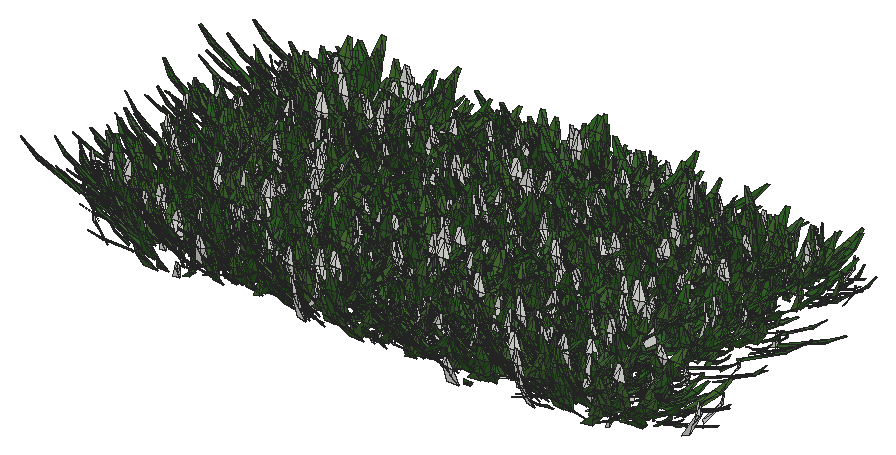
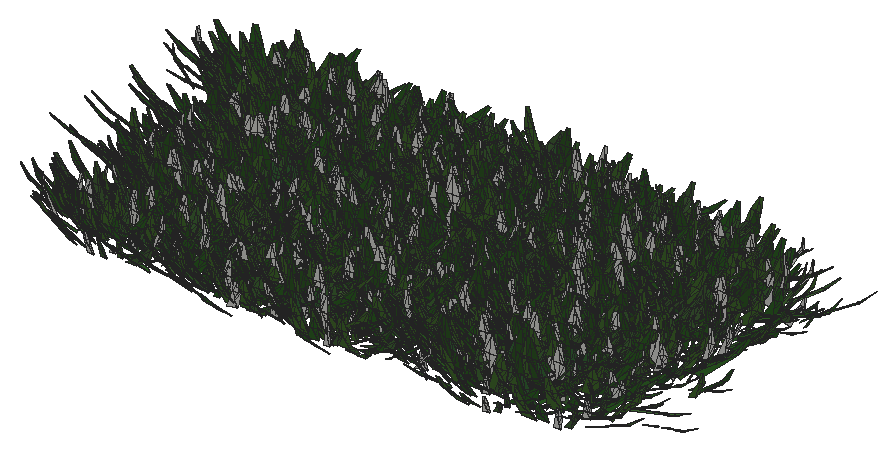
# SketchUp Ruby script. Lengths in inches.
U = 1.inch
M = Sketchup.active_model
def pt(a) = Geom::Point3d.new(a.map { |v| v * U })
def face(e, loops, mat)
  f = e.add_face(loops[0].map { |a| pt(a) })
  loops[1..].each { |l| e.add_face(l.map { |a| pt(a) }).erase! }
  f.material = f.back_material = mat if mat
  f
end
# faces: each face lists its corners as indices into pts; further lists are holes
def faces(e, pts, list, mat = nil) = list.each { |f| face(e, (f[0].is_a?(Array) ? f : [f]).map { |l| l.map { |i| pts[i] } }, mat) }
# xy, xz, yz: faces in a plane at the given z, y or x. An outline is a flat list of corners, or four numbers for a rectangle; further outlines are holes
def ring(l) = l.size == 4 ? [[l[0], l[1]], [l[2], l[1]], [l[2], l[3]], [l[0], l[3]]] : l.each_slice(2).to_a
def flat(e, list, mat, &to3) = list.each { |f| face(e, (f[0].is_a?(Array) ? f : [f]).map { |l| ring(l).map { |u, v| to3.(u, v) } }, mat) }
def xy(e, z, list, mat = nil) = flat(e, list, mat) { |x, y| [x, y, z] }
def xz(e, y, list, mat = nil) = flat(e, list, mat) { |x, z| [x, y, z] }
def yz(e, x, list, mat = nil) = flat(e, list, mat) { |y, z| [x, y, z] }
def lines(e, pts, list) = list.each { |a, b| e.add_line(pt(pts[a]), pt(pts[b])) }
# prism: a flat outline (further loops are holes) pulled along v
def prism(e, loops, v, mat = nil)
  f = face(e, loops, mat); d = Geom::Vector3d.new(v.map { |x| x * U })
  f.pushpull(f.normal.samedirection?(d) ? d.length : -d.length)
end
def box(e, o, s, mat = nil) = prism(e, [[o, [o[0] + s[0], o[1], o[2]], [o[0] + s[0], o[1] + s[1], o[2]], [o[0], o[1] + s[1], o[2]]]], [0, 0, s[2]], mat)
def at(x, y, z, deg = 0) = Geom::Transformation.translation(pt([x, y, z])) * Geom::Transformation.rotation(ORIGIN, Z_AXIS, deg.degrees)
def axes(o, x, y, z) = Geom::Transformation.new([*x, 0, *y, 0, *z, 0, *pt(o).to_a, 1])
def part(name) = M.definitions.add(name)
# library, detail: a bought-in or finely detailed component or shape, given as its bounding box
def library(name, o, s) = part(name).tap { |d| box(d.entities, o, s) }
def detail(e, o, s) = box(e.add_group.entities, o, s)
def put(e, d, t, mat = nil) = e.add_instance(d, t).tap { |i| i.material = mat if mat }
def group(e, t, mat = nil) = e.add_group.tap { |g| g.transformation = t; g.material = mat if mat }.entities
root = M.entities
M.materials.add("Material82").color = [68, 110, 58]
M.materials.add("Material83").color = [48, 90, 38]
M.materials.add("Material84").color = [68, 110, 48]
M.materials.add("Material85").color = [48, 90, 48]
M.materials.add("Material86").color = [58, 110, 58]
M.materials.add("Material87").color = [58, 90, 38]
M.materials.add("Material88").color = [68, 100, 58]
M.materials.add("Material89").color = [48, 100, 38]
c1 = part("grass00")
p = [[-0.6875,0.15,0],[-0.56,0.08,5.52],[-0.04,0.03,2.76],[0.48,-0.02,0],[0.35,-0.02,5.52],[-0.1,-0.14,5.52],
  [-0.12,0.65,8.37],[-0.42,0.65,8.37]]
faces(c1.entities,p,[[0,1,2,3],[3,2,4],[1,5,2],[5,4,2],[1,6,5],[4,5,6],[7,6,1]])
c2 = part("Group16\#1")
put(c2.entities,c1,axes([1.44,-0.61,-0.01],[0.05352,0.12609,0],[-0.10704,0.04543,0.07239],[0.06664,-0.02828,0.11628]),"Material85")
put(c2.entities,c1,axes([0.76,-0.15,-0.01],[0.04676,0.24062,0],[-0.23162,0.04501,0.06642],[0.0652,-0.01267,0.23595]),"Material82")
put(c2.entities,c1,axes([0.79,0.01,-0.01],[-0.00606,0.34651,0],[-0.34381,-0.00602,0.0432],[0.04319,0.00076,0.34386]))
put(c2.entities,c1,axes([1,0.23,-0.01],[-0.07192,0.31144,0],[-0.28722,-0.06632,0.1236],[0.12043,0.02781,0.29478]),"Material84")
put(c2.entities,c1,axes([1.66,0.77,-0.01],[-0.13828,0.29651,0],[-0.21551,-0.1005,0.22471],[0.20365,0.09498,0.23779]),"Material89")
put(c2.entities,c1,axes([0.6875,0.52,-0.01],[-0.18126,0.24051,0],[-0.22746,-0.17142,0.09788],[0.07817,0.05891,0.28481]),"Material84")
put(c2.entities,c1,axes([0.68,0.78,-0.01],[-0.215,0.18688,0],[-0.12385,-0.14248,0.21334],[0.13995,0.16101,0.18878]),"Material82")
put(c2.entities,c1,axes([0.56,1,-0.01],[-0.13756,0.07624,0],[-0.06159,-0.11112,0.0927],[0.04494,0.08108,0.12705]),"Material84")
put(c2.entities,c1,axes([0.2,0.64,-0.01],[-0.23729,0.07254,0],[-0.05711,-0.18681,0.153],[0.04473,0.14632,0.19535]),"Material89")
put(c2.entities,c1,axes([0.0625,0.72,-0.01],[-0.28874,0.02525,0],[-0.02179,-0.24916,0.14647],[0.01276,0.14591,0.25012]),"Material82")
put(c2.entities,c1,axes([-0.08,0.62,-0.01],[-0.34089,-0.04187,0],[0.03255,-0.26504,0.216],[-0.02633,0.21439,0.26703]),"Material89")
put(c2.entities,c1,axes([-0.34,0.98,-0.01],[-0.14314,-0.0493,0],[0.04397,-0.12769,0.06843],[-0.02228,0.0647,0.13505]),"Material89")
put(c2.entities,c1,axes([-0.87,1.45,-0.01],[-0.23488,-0.14114,0],[0.13761,-0.22901,0.06087],[-0.03135,0.05217,0.26717]))
put(c2.entities,c1,axes([-0.72,0.77,-0.01],[-0.14208,-0.13251,0],[0.07209,-0.0773,0.16301],[-0.11118,0.11922,0.1057]),"Material89")
put(c2.entities,c1,axes([-0.62,0.43,-0.01],[-0.14845,-0.21203,0],[0.18654,-0.13061,0.12304],[-0.10079,0.07057,0.22772]),"Material82")
put(c2.entities,c1,axes([-0.68,0.29,-0.01],[-0.13639,-0.32136,0],[0.31723,-0.13464,0.05579],[-0.05136,0.0218,0.34462]),"Material83")
put(c2.entities,c1,axes([-0.64,0.125,-0.01],[-0.0458,-0.23569,0],[0.22124,-0.043,0.08276],[-0.08124,0.01579,0.22538]),"Material86")
put(c2.entities,c1,axes([-1.6,-0.03,-0.01],[0.00576,-0.32897,0],[0.27526,0.00482,0.18018],[-0.18015,-0.00315,0.2753]),"Material84")
put(c2.entities,c1,axes([-1.36,-0.31,-0.01],[0.05718,-0.24765,0],[0.18172,0.04196,0.17267],[-0.16825,-0.03885,0.1865]),"Material89")
put(c2.entities,c1,axes([-1.54,-0.72,-0.01],[0.06537,-0.14017,0],[0.13555,0.06321,0.03939],[-0.0357,-0.01665,0.14956]))
put(c2.entities,c1,axes([-1.19,-0.9,-0.01],[0.09597,-0.12735,0],[0.11214,0.08451,0.07557],[-0.06035,-0.04548,0.14042]),"Material88")
put(c2.entities,c1,axes([-0.47,-0.54,-0.01],[0.11588,-0.10072,0],[0.0618,0.0711,0.12124],[-0.07953,-0.0915,0.0942]))
put(c2.entities,c1,axes([-0.47,-0.84,-0.01],[0.11927,-0.0661,0],[0.06603,0.11913,0.00646],[-0.00313,-0.00565,0.13621]),"Material84")
put(c2.entities,c1,axes([-0.38,-1.24,-0.01],[0.28037,-0.08571,0],[0.0618,0.20215,0.20315],[-0.05939,-0.19428,0.21139]),"Material88")
put(c2.entities,c1,axes([-0.06,-0.66,-0.01],[0.22719,-0.01987,0],[0.01247,0.14255,0.17758],[-0.01547,-0.17691,0.1431]),"Material87")
put(c2.entities,c1,axes([0.11,-0.89,-0.01],[0.14882,0.01828,0],[-0.01058,0.08611,0.12229],[0.01491,-0.12138,0.08676]),"Material85")
put(c2.entities,c1,axes([0.25,-0.72,-0.01],[0.20481,0.07053,0],[-0.06206,0.18022,0.10291],[0.03351,-0.0973,0.1906]),"Material85")
put(c2.entities,c1,axes([0.85,-1.42,-0.01],[0.16481,0.09904,0],[-0.09472,0.15762,0.05616],[0.02893,-0.04814,0.18389]),"Material84")
put(c2.entities,c1,axes([1.01,-1.09,-0.01],[0.21858,0.20385,0],[-0.17495,0.1876,0.15339],[0.10462,-0.11218,0.25652]),"Material89")
put(c2.entities,c1,axes([1.01,-0.71,-0.01],[0.08733,0.12473,0],[-0.06445,0.04512,0.13037],[0.1068,-0.07477,0.07867]),"Material85")
c3 = part("Group15\#1")
put(c3.entities,c2,at(0,0,0))
c4 = part("3darcstudiotree_grass00\#1")
put(c4.entities,c3,at(0,0,0))
put(root,c4,axes([1698.13,360.98,-34.17],[-3.55958,-1.14913,0],[2.41323,-1.16263,-0.04086],[0.15936,-0.07677,1.75811]))
put(root,c4,axes([1698.43,351.33,-34.17],[-0.43927,-1.56699,0],[3.3973,-0.14812,-0.00454],[0.02991,-0.0013,1.6986]))
put(root,c4,axes([1698.77,345.77,-34.17],[-1.97176,-1.44506,0],[3.679,-0.78074,-0.04084],[0.18174,-0.03857,1.58232]))
put(root,c4,axes([1698.59,344.4375,-34.17],[-3.51315,0.12017,0],[-0.35069,-1.59447,-0.04163],[-0.0224,-0.10183,1.89396]))
put(root,c4,axes([1699.35,359.99,-34.17],[-1.25158,-1.24653,0],[3.09013,-0.48255,-0.01359],[0.08484,-0.01325,1.67314]))
put(root,c4,axes([1698.75,366.44,-34.17],[-2.97894,1.37787,0],[-2.78264,-0.93567,-0.01811],[-0.06538,-0.02199,1.30017]))
put(root,c4,axes([1699.02,354.66,-34.17],[3.2382,0.426,0],[-1.27463,1.50694,-0.00681],[-0.01361,0.01609,1.90695]))
put(root,c4,axes([1700.85,370.73,-34.17],[0.12202,-1.72029,0],[4.34373,0.04792,-0.00421],[0.02346,0.00026,1.81536]))
put(root,c4,axes([1699.33,352.6875,-34.17],[3.02682,0.57541,0],[-1.48298,1.21327,-0.04063],[-0.10557,0.08637,1.53169]))
put(root,c4,axes([1699.47,347.92,-34.17],[-0.79088,1.37944,0],[-4.55872,-0.4065,-0.04071],[-0.16308,-0.01454,1.43871]))
put(root,c4,axes([1701.78,368.09,-34.17],[1.28722,-1.76401,0],[4.46987,0.50729,-0.04991],[0.26732,0.03034,1.94306]))
put(root,c4,axes([1700.9,357.65,-34.17],[3.67827,0.2088,0],[-0.57305,1.57009,-0.04848],[-0.0346,0.09479,1.51023]))
put(root,c4,axes([1702,364.37,-34.17],[1.80491,-1.57701,0],[4.14536,0.7379,-0.03311],[0.16907,0.03009,1.9099]))
put(root,c4,axes([1701.94,341.82,-34.17],[-0.04598,1.31401,0],[-3.68449,-0.02005,-0.02407],[-0.13013,-0.00071,1.49365]))
put(root,c4,axes([1704.48,349.01,-34.17],[0.08239,-1.33128,0],[3.65037,0.03514,-0.00377],[0.02295,0.00022,1.66719]))
put(root,c4,axes([1704.05,367.54,-34.17],[-1.91663,1.65988,0],[-3.0087,-0.54032,-0.04508],[-0.21948,-0.03942,1.32557]))
put(root,c4,axes([1704.23,357.93,-34.17],[-2.0309,1.41107,0],[-3.96455,-0.88745,-0.03094],[-0.10652,-0.02384,1.35284]))
put(root,c4,axes([1704.05,359.23,-34.17],[3.97679,-0.10087,0],[0.2922,1.7917,-0.04097],[0.01281,0.07857,1.66267]))
put(root,c4,axes([1704.71,365.41,-34.17],[2.96266,-0.9536,0],[2.21709,1.07131,-0.03627],[0.16479,0.07963,1.88825]))
put(root,c4,axes([1705.87,350.52,-34.17],[-2.64678,-1.36079,0],[3.05956,-0.92555,-0.03114],[0.16031,-0.04849,1.87535]))
put(root,c4,axes([1704.4,353.46,-34.17],[1.36747,1.27936,0],[-3.91602,0.651,-0.04214],[-0.23603,0.03924,1.93625]))
put(root,c4,axes([1706.28,372.32,-34.17],[-0.46652,-1.63259,0],[3.80254,-0.169,-0.02839],[0.12966,-0.00576,1.31807]))
put(root,c4,axes([1706.08,362.02,-34.17],[-2.52022,1.35688,0],[-2.71694,-0.78485,-0.02032],[-0.10759,-0.03108,1.65635]))
put(root,c4,axes([1706.72,342.15,-34.17],[-3.93546,0.24929,0],[-0.63824,-1.56709,-0.04907],[-0.04216,-0.10352,1.63442]))
put(root,c4,axes([1705.48,339.35,-34.17],[-0.1961,1.67231,0],[-3.9427,-0.07191,-0.00948],[-0.04368,-0.0008,1.36423]))
put(root,c4,axes([1705.6,363.85,-34.17],[0.89151,1.73156,0],[-4.53511,0.36315,-0.02679],[-0.1364,0.01092,1.80175]))
put(root,c4,axes([1706.1875,343.8125,-34.17],[3.29656,-0.16392,0],[0.52833,1.6525,-0.05027],[0.03097,0.09687,1.55905]))
put(root,c4,axes([1707.03,355.55,-34.17],[2.92684,-0.73502,0],[1.91435,1.18558,-0.0345],[0.12831,0.07947,1.8497]))
put(root,c4,axes([1707.23,346.87,-34.17],[0.10092,1.39888,0],[-4.08431,0.04583,-0.02239],[-0.13434,0.00151,1.83839]))
put(root,c4,axes([1707.31,370.06,-34.17],[-0.46714,1.44095,0],[-4.49775,-0.22678,-0.0277],[-0.15196,-0.00766,1.87956]))
put(root,c4,axes([1709.33,360.11,-34.17],[-2.63576,-1.28026,0],[3.53005,-1.13032,-0.02494],[0.11128,-0.03563,1.95866]))
put(root,c4,axes([1709.03,370.33,-34.17],[-0.06008,-1.38054,0],[4.09358,-0.02771,-0.0405],[0.24938,-0.00169,1.89003]))
put(root,c4,axes([1710.19,362.39,-34.17],[-2.86404,-0.64452,0],[1.81455,-1.25407,-0.04344],[0.15373,-0.10625,1.9596]))
put(root,c4,axes([1710.43,350.28,-34.17],[-1.66133,-1.5225,0],[4.09169,-0.6944,-0.04688],[0.21591,-0.03664,1.67419]))
put(root,c4,axes([1710.36,356.79,-34.17],[-3.61877,0.99301,0],[-2.17277,-1.23149,-0.01001],[-0.02667,-0.01512,1.32974]))
put(root,c4,axes([1711.375,368.29,-34.17],[-0.34586,-1.45501,0],[4.09876,-0.15153,-0.00863],[0.04038,-0.00149,1.44957]))
put(root,c4,axes([1711.95,355.14,-34.17],[-1.55676,-1.64059,0],[4.33421,-0.63965,-0.05081],[0.20494,-0.03024,1.49393]))
put(root,c4,axes([1710.55,365.77,-34.17],[4.37611,-0.60729,0],[1.31361,1.47222,-0.0057],[0.0109,0.01221,1.70987]))
put(root,c4,axes([1712.45,343.71,-34.17],[-3.927,-0.17218,0],[0.45946,-1.62986,-0.05312],[0.03146,-0.11159,1.67036]))
put(root,c4,axes([1711.36,341.7,-34.17],[4.2823,-0.66393,0],[1.32307,1.32724,-0.00849],[0.02062,0.02068,1.79934]))
put(root,c4,axes([1712.68,363.99,-34.17],[-3.78815,1.05417,0],[-2.08305,-1.1642,0],[-0.00001,-0.00001,1.91868]))
put(root,c4,axes([1711.93,340.27,-34.17],[3.14187,0.39177,0],[-1.17778,1.46906,-0.04459],[-0.07661,0.09555,1.66873]))
put(root,c4,axes([1712.84,346.79,-34.17],[-2.14427,1.00131,0],[-3.09998,-1.03248,-0.03207],[-0.1604,-0.05342,1.99077]))
put(root,c4,axes([1713.02,348.81,-34.17],[-3.03453,1.36043,0],[-3.50876,-1.21725,-0.06393],[-0.1925,-0.06678,1.40472]))
put(root,c4,axes([1712.85,352.39,-34.17],[4.55933,-0.17295,0],[0.45061,1.84755,-0.06081],[0.02387,0.09789,1.44654]))
put(root,c4,axes([1714.71,367.64,-34.17],[-0.03672,-1.35909,0],[4.67682,-0.01965,-0.05216],[0.20276,-0.00085,1.36288]))
put(root,c4,axes([1714.8125,353.11,-34.17],[0.13892,-1.80916,0],[4.0915,0.04886,-0.01983],[0.09749,0.00116,1.50947]))
put(root,c4,axes([1715.21,357.1,-34.17],[-3.75519,-1.14447,0],[2.68213,-1.36874,-0.06061],[0.1619,-0.08262,1.43628]))
put(root,c4,axes([1714.73,369.82,-34.17],[-0.54027,-1.6401,0],[3.32557,-0.17038,-0.04034],[0.23473,-0.01203,1.47504]))
put(root,c4,axes([1714.97,365.63,-34.17],[-3.58356,0.46021,0],[-1.0679,-1.2933,-0.04555],[-0.08783,-0.10637,1.60995]))
put(root,c4,axes([1715.44,343.83,-34.17],[-3.8661,0.57248,0],[-1.34665,-1.41442,-0.01194],[-0.02505,-0.02631,1.71307]))
put(root,c4,axes([1715.64,351.27,-34.17],[-3.59396,1.08002,0],[-2.30452,-1.19271,-0.04347],[-0.15376,-0.07958,1.66314]))
put(root,c4,axes([1716.42,340.48,-34.17],[-3.24117,-0.71309,0],[1.62667,-1.14993,-0.00653],[0.01841,-0.01301,1.4475]))
put(root,c4,axes([1715.13,363.49,-34.17],[-0.46786,1.28327,0],[-3.81344,-0.21623,-0.00494],[-0.02392,-0.00136,1.4129]))
put(root,c4,axes([1716.92,346.46,-34.17],[0.52643,-1.67667,0],[4.29673,0.20982,-0.00236],[0.01155,0.00056,1.5989]))
put(root,c4,axes([1715.86,348.07,-34.17],[4.26757,-0.1267,0],[0.26808,1.40432,-0.02417],[0.01226,0.06424,1.80918]))
put(root,c4,axes([1717.47,359.21,-34.17],[-4.03193,0.12785,0],[-0.33897,-1.66251,-0.04274],[-0.01416,-0.06944,1.31001]))
put(root,c4,axes([1716.1,361.24,-34.17],[2.51292,1.08795,0],[-3.26468,1.1728,-0.05824],[-0.20485,0.07359,1.57486]))
put(root,c4,axes([1716.59,341.95,-34.17],[2.57949,0.81299,0],[-2.19489,1.0831,-0.04441],[-0.18645,0.09201,1.772]))
put(root,c4,axes([1717.76,354.82,-34.17],[1.65411,1.32331,0],[-4.02119,0.78176,-0.01549],[-0.05875,0.01142,1.42146]))
put(root,c4,axes([1720.5,341.48,-34.17],[-1.99996,-1.21087,0],[3.64955,-0.93751,-0.00487],[0.02184,-0.00561,1.74651]))
put(root,c4,axes([1720.74,344.25,-34.17],[0.76825,-1.34447,0],[4.07723,0.36235,-0.02216],[0.10533,0.00936,1.52603]))
put(root,c4,axes([1721.66,353.16,-34.17],[-0.47602,-1.5827,0],[4.1601,-0.1946,-0.02638],[0.12052,-0.00564,1.44452]))
put(root,c4,axes([1720.96,361.75,-34.17],[-1.67139,1.30839,0],[-3.46219,-0.68786,-0.03585],[-0.17478,-0.03472,1.58646]))
put(root,c4,axes([1721.55,368.33,-34.17],[-3.50073,0.942,0],[-2.16331,-1.25037,-0.04776],[-0.1565,-0.09046,1.6727]))
put(root,c4,axes([1720.9,360.04,-34.17],[3.80678,-0.63656,0],[1.53404,1.42681,-0.02583],[0.05775,0.05372,1.68703]))
put(root,c4,axes([1721.85,354.56,-34.17],[3.46257,-0.87441,0],[2.25752,1.39035,-0.00312],[0.00811,0.00499,1.51309]))
put(root,c4,axes([1721.48,357.61,-34.17],[4.45522,-0.42871,0],[0.88291,1.42703,-0.01844],[0.02851,0.04608,1.82062]))
put(root,c4,axes([1722.52,348.22,-34.17],[2.70908,-1.29001,0],[3.26836,1.0675,-0.01649],[0.07179,0.02345,1.79785]))
put(root,c4,axes([1723.25,370.96,-34.17],[-1.99014,-1.36063,0],[3.61455,-0.82226,-0.05686],[0.20653,-0.04698,1.31145]))
put(root,c4,axes([1722.92,366.26,-34.17],[1.2093,-1.57862,0],[4.10109,0.48862,-0.03916],[0.21176,0.02523,1.81408]))
put(root,c4,axes([1721.46,372.33,-34.17],[2.22707,1.32751,0],[-3.83725,1.00121,-0.02773],[-0.10131,0.02643,1.51065]))
put(root,c4,axes([1722.4375,345.68,-34.17],[3.29328,0.79365,0],[-2.38723,1.54066,-0.04231],[-0.12354,0.07973,1.92144]))
put(root,c4,axes([1724.15,351.2,-34.17],[-4.33123,0.18779,0],[-0.372,-1.33439,-0.04038],[-0.02759,-0.09898,1.5952]))
put(root,c4,axes([1723.8,340.03,-34.17],[-2.43738,1.19248,0],[-2.72185,-0.86527,-0.02131],[-0.12,-0.03815,1.8955]))
put(root,c4,axes([1723.74,364.4,-34.17],[-1.08989,1.28976,0],[-3.11811,-0.40981,-0.02384],[-0.1661,-0.02183,1.80943]))
put(root,c4,axes([1725.64,372.52,-34.17],[0.31301,-1.31124,0],[3.5948,0.13346,-0.01523],[0.11152,0.00414,1.99019]))
put(root,c4,axes([1726.2,345.68,-34.17],[-3.40339,-1.11564,0],[2.13204,-1.01156,-0.01701],[0.08509,-0.04037,1.95649]))
put(root,c4,axes([1726.56,358.8125,-34.17],[-3.55731,-0.39699,0],[0.91028,-1.26863,-0.03071],[0.04629,-0.06451,1.38702]))
put(root,c4,axes([1726.07,353.5,-34.17],[1.53941,-1.17663,0],[3.76142,0.76538,-0.04957],[0.23972,0.04878,1.72633]))
put(root,c4,axes([1726.26,351.05,-34.17],[1.91221,-1.68967,0],[4.00415,0.70478,-0.04062],[0.20203,0.03556,1.79015]))
put(root,c4,axes([1726.13,357.86,-34.17],[3.14616,-0.46124,0],[1.36147,1.44435,-0.02775],[0.06352,0.06739,1.92398]))
put(root,c4,axes([1727.52,366.51,-34.17],[-0.59398,-1.49967,0],[3.68059,-0.22673,-0.04759],[0.22724,-0.014,1.34947]))
put(root,c4,axes([1728.37,355.07,-34.17],[1.44153,-1.60776,0],[3.23959,0.45176,-0.02361],[0.11408,0.01591,1.32009]))
put(root,c4,axes([1727.8,349.43,-34.17],[-0.86085,1.83609,0],[-4.61027,-0.33618,-0.00297],[-0.01572,-0.00115,1.8915]))
put(root,c4,axes([1727.72,342.07,-34.17],[2.91821,1.08875,0],[-2.82314,1.17688,-0.00432],[-0.01382,0.00576,1.43292]))
put(root,c4,axes([1728.98,370.32,-34.17],[3.48292,-0.82099,0],[2.25154,1.48559,-0.05659],[0.14545,0.09597,1.64805]))
put(root,c4,axes([1728.4375,339.77,-34.17],[4.39717,0.52423,0],[-1.00944,1.31686,-0.04581],[-0.07981,0.10411,1.57403]))
put(root,c4,axes([1728.41,368.5,-34.17],[3.42406,1.01361,0],[-2.506,1.31662,-0.02233],[-0.08435,0.04432,1.9689]))
put(root,c4,axes([1729.13,361.89,-34.17],[-2.64058,1.54622,0],[-3.55505,-0.94424,-0.0002],[-0.001,-0.00026,1.96126]))
put(root,c4,axes([1729.47,363.25,-34.17],[4.33275,-0.34682,0],[0.77843,1.5125,-0.04034],[0.04996,0.09707,1.82611]))
put(root,c4,axes([1729.4375,345.04,-34.17],[3.65442,0.79234,0],[-1.92667,1.38205,-0.0244],[-0.05154,0.03697,1.31386]))
put(root,c4,axes([1731.86,364.07,-34.17],[-4.47242,-0.43212,0],[1.12449,-1.81009,-0.038],[0.04833,-0.0778,1.89315]))
put(root,c4,axes([1732.93,357.43,-34.17],[2.42149,-1.19086,0],[3.28427,1.03866,-0.04277],[0.16953,0.05361,1.60323]))
put(root,c4,axes([1733.89,346.67,-34.17],[-4.5051,-0.1347,0],[0.33952,-1.76605,-0.05601],[0.0175,-0.09103,1.39118]))
put(root,c4,axes([1734.02,350.83,-34.17],[-3.05686,-1.19982,0],[3.00062,-1.189,-0.05331],[0.20258,-0.08027,1.71744]))
put(root,c4,axes([1734.02,348.13,-34.17],[0.58993,-1.49665,0],[4.0908,0.25078,-0.01704],[0.09795,0.00601,1.80481]))
put(root,c4,axes([1732.57,343.77,-34.17],[0.93986,1.81776,0],[-4.11362,0.3308,-0.03996],[-0.17618,0.01417,1.416]))
put(root,c4,axes([1732.57,372.17,-34.17],[1.86,1.67689,0],[-3.22779,0.55683,-0.02724],[-0.14202,0.0245,1.50258]))
put(root,c4,axes([1732.86,355.82,-34.17],[3.80375,0.01195,0],[-0.02861,1.41659,-0.01492],[-0.00081,0.04025,1.84219]))
put(root,c4,axes([1732.89,340.18,-34.17],[3.00521,0.63807,0],[-1.62064,1.18715,-0.02125],[-0.05194,0.03805,1.32121]))
put(root,c4,axes([1733.92,365.9375,-34.17],[-1.91722,1.31385,0],[-4.0358,-0.91594,-0.03664],[-0.12047,-0.02734,1.3241]))
put(root,c4,axes([1734.16,359.45,-34.17],[4.38931,-0.45982,0],[1.18067,1.75286,-0.06211],[0.07411,0.11002,1.60192]))
put(root,c4,axes([1733.9,371.3,-34.17],[3.90875,0.99817,0],[-2.33451,1.4218,-0.02279],[-0.07245,0.04412,1.88252]))
put(root,c4,axes([1734.47,361.58,-34.17],[4.17909,0.84834,0],[-2.02565,1.55199,-0.04224],[-0.09233,0.07074,1.58426]))
put(root,c4,axes([1734.89,341.35,-34.17],[3.56991,0.07978,0],[-0.21949,1.52742,-0.02759],[-0.00848,0.05902,1.57942]))
put(root,c4,axes([1736.69,354.51,-34.17],[-4.32084,-0.18562,0],[0.42888,-1.55273,-0.0047],[0.00255,-0.00922,1.4854]))
put(root,c4,axes([1735.13,368.89,-34.17],[0.16976,1.81896,0],[-4.60297,0.06681,-0.03073],[-0.13236,0.00192,1.48809]))
put(root,c4,axes([1737.06,371.02,-34.17],[-3.5417,-0.59044,0],[1.62012,-1.51145,-0.0473],[0.08471,-0.07903,1.43445]))
put(root,c4,axes([1735.25,353.31,-34.17],[4.0668,0.76332,0],[-1.54133,1.27718,-0.01473],[-0.03515,0.02913,1.49308]))
put(root,c4,axes([1736.84,357.81,-34.17],[-3.98791,0.79031,0],[-1.65069,-1.29546,-0.0516],[-0.1637,-0.12847,1.94674]))
put(root,c4,axes([1737.37,361.73,-34.17],[-3.83726,0.13979,0],[-0.31883,-1.36117,-0.04806],[-0.027,-0.11528,1.58689]))
put(root,c4,axes([1738.2,350.08,-34.17],[-3.41944,0.15794,0],[-0.40533,-1.36487,-0.03745],[-0.0251,-0.08453,1.50509]))
put(root,c4,axes([1736.91,344.37,-34.17],[0.51016,1.70246,0],[-4.00788,0.18679,-0.00527],[-0.02601,0.00121,1.50433]))
put(root,c4,axes([1737.38,372.3,-34.17],[3.76255,0.21279,0],[-0.50611,1.39184,-0.02285],[-0.01632,0.04489,1.34478]))
put(root,c4,axes([1738.85,340.09,-34.17],[-4.15336,0.88478,0],[-2.07336,-1.51373,-0.03525],[-0.06704,-0.04895,1.3087]))
put(root,c4,axes([1739.02,347.01,-34.17],[1.23783,-1.57966,0],[3.18362,0.388,-0.00928],[0.06663,0.00812,1.87692]))
put(root,c4,axes([1737.85,359.74,-34.17],[4.18297,0.824,0],[-1.87304,1.47883,-0.04234],[-0.08644,0.06825,1.4356]))
put(root,c4,axes([1740.7,367.52,-34.17],[-4.24589,-0.20577,0],[0.52914,-1.69815,-0.04768],[0.02678,-0.08595,1.49744]))
put(root,c4,axes([1739.22,352.74,-34.17],[0.88024,1.52698,0],[-4.39329,0.39388,-0.06457],[-0.26955,0.02417,1.44574]))
put(root,c4,axes([1740.25,341.93,-34.17],[2.74133,-1.23391,0],[3.31507,1.14547,-0.04981],[0.18948,0.06547,1.67091]))
put(root,c4,axes([1739.35,365.63,-34.17],[3.13752,1.05459,0],[-2.29496,1.06192,-0.00613],[-0.02513,0.01163,1.67562]))
put(root,c4,axes([1740.21,347.84,-34.17],[1.5924,1.20755,0],[-3.44476,0.70651,-0.03549],[-0.1652,0.03388,1.52707]))
put(root,c4,axes([1740,364.09,-34.17],[1.54833,1.52017,0],[-4.09421,0.64856,-0.00669],[-0.03642,0.00577,1.94122]))
put(root,c4,axes([1742.67,363.53,-34.17],[-0.04856,-1.33378,0],[4.56796,-0.02587,-0.06189],[0.3016,-0.00171,1.66883]))
put(root,c4,axes([1743.9,370.44,-34.17],[-4.54384,0.18076,0],[-0.35947,-1.40543,-0.00469],[-0.00344,-0.01343,1.96044]))
put(root,c4,axes([1744.24,342.31,-34.17],[-3.26554,0.66263,0],[-1.53451,-1.17616,-0.01759],[-0.06154,-0.04717,1.92222]))
put(root,c4,axes([1744.03,354.88,-34.17],[2.51439,-1.31879,0],[3.78,1.12088,-0.05965],[0.2657,0.07879,1.97549]))
put(root,c4,axes([1744.8125,356.6,-34.17],[-0.70547,-1.57622,0],[3.40493,-0.23702,-0.01992],[0.12135,-0.00845,1.60321]))
put(root,c4,axes([1743.24,350.71,-34.17],[4.47557,0.19067,0],[-0.50576,1.84642,-0.03307],[-0.01603,0.05854,1.59331]))
put(root,c4,axes([1743.67,366.21,-34.17],[0.58274,1.76141,0],[-3.38049,0.17394,-0.03746],[-0.24477,0.01259,1.68385]))
put(root,c4,axes([1744.35,347.91,-34.17],[-3.09447,0.74267,0],[-2.17746,-1.41107,-0.01391],[-0.03982,-0.0258,1.7292]))
put(root,c4,axes([1744.57,352.47,-34.17],[2.464,-1.39681,0],[2.85004,0.78193,-0.02795],[0.16419,0.04505,1.86246]))
put(root,c4,axes([1744.47,359.98,-34.17],[-1.84293,1.54258,0],[-3.69335,-0.68627,-0.00165],[-0.00726,-0.00135,1.48801]))
put(root,c4,axes([1746.0625,343.68,-34.17],[-4.60496,-0.17881,0],[0.42059,-1.68464,-0.00134],[0.00055,-0.00219,1.33719]))
put(root,c4,axes([1745.64,346.44,-34.17],[2.67997,-1.42027,0],[3.59345,1.05458,-0.05496],[0.18586,0.05455,1.41537]))
put(root,c4,axes([1745.83,361.42,-34.17],[0.63899,1.37464,0],[-4.27438,0.30902,-0.00804],[-0.04314,0.00312,1.77733]))
put(root,c4,axes([1746.08,368.8,-34.17],[1.87438,1.56788,0],[-3.52749,0.65588,-0.03917],[-0.21764,0.04047,1.79585]))
put(root,c4,axes([1748.59,343.99,-34.17],[-1.02752,-1.39563,0],[3.42384,-0.39205,-0.00444],[0.02976,-0.00341,1.86591]))
put(root,c4,axes([1748.02,363.61,-34.17],[1.33366,-1.36849,0],[3.54112,0.53673,-0.03841],[0.22056,0.03343,1.74904]))
put(root,c4,axes([1748.49,372.1875,-34.17],[-1.96103,-1.06216,0],[3.43549,-0.98649,-0.06067],[0.27868,-0.08002,1.80988]))
put(root,c4,axes([1748.38,348.42,-34.17],[-3.04968,0.59415,0],[-1.75652,-1.40223,-0.03032],[-0.06781,-0.05413,1.50108]))
put(root,c4,axes([1748.97,340.7,-34.17],[-2.6125,1.23987,0],[-2.75746,-0.90365,-0.04997],[-0.20997,-0.06881,1.46822]))
put(root,c4,axes([1748.69,347,-34.17],[-0.25979,1.36498,0],[-3.68566,-0.1091,-0.02554],[-0.15097,-0.00447,1.64241]))
put(root,c4,axes([1750.45,352.27,-34.17],[-4.34871,0.30764,0],[-0.79873,-1.75601,-0.00093],[-0.00077,-0.00169,1.58752]))
put(root,c4,axes([1749.27,342.48,-34.17],[3.80887,0.06416,0],[-0.18164,1.67717,-0.01987],[-0.00391,0.03608,1.47043]))
put(root,c4,axes([1749.29,355.03,-34.17],[4.17174,-0.07865,0],[0.15922,1.3134,-0.03217],[0.01066,0.0879,1.73328]))
put(root,c4,axes([1749.49,357.09,-34.17],[3.86863,-0.34225,0],[0.73265,1.28801,-0.00297],[0.00437,0.00768,1.68702]))
put(root,c4,axes([1749.69,366.9,-34.17],[3.26947,0.70015,0],[-1.66816,1.21153,-0.03457],[-0.12105,0.08791,1.92264]))
put(root,c4,axes([1750.26,351.22,-34.17],[-1.46805,1.46647,0],[-4.14161,-0.64484,-0.02576],[-0.10998,-0.01712,1.53201]))
put(root,c4,axes([1750.34,359.15,-34.17],[4.25624,-0.01859,0],[0.03959,1.4097,-0.01976],[0.00112,0.03979,1.36845]))
put(root,c4,axes([1750.57,370.34,-34.17],[2.49415,0.97261,0],[-2.31115,0.92177,-0.02576],[-0.13853,0.05525,1.88472]))
put(root,c4,axes([1751.79,360.97,-34.17],[-2.30622,1.23379,0],[-2.8482,-0.82802,-0.0238],[-0.11552,-0.03358,1.59896]))
put(root,c4,axes([1751.42,369.02,-34.17],[1.30118,1.34593,0],[-3.49846,0.52602,-0.01397],[-0.0708,0.01064,1.52193]))
put(root,c4,axes([1753.99,342.78,-34.17],[-2.87014,-1.48867,0],[3.23188,-0.96911,-0.02],[0.09309,-0.02792,1.779]))
put(root,c4,axes([1753.77,344.18,-34.17],[-0.3493,-1.81077,0],[4.63308,-0.139,-0.05882],[0.26935,-0.00808,1.5994]))
